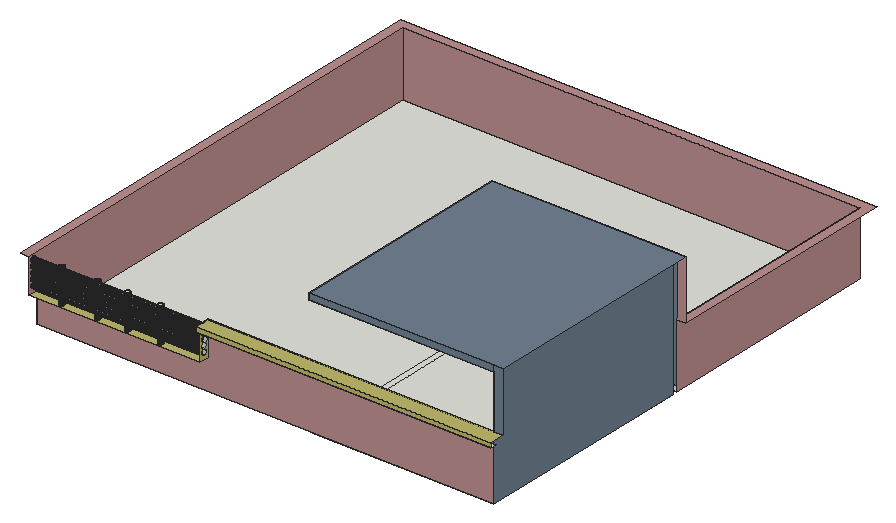
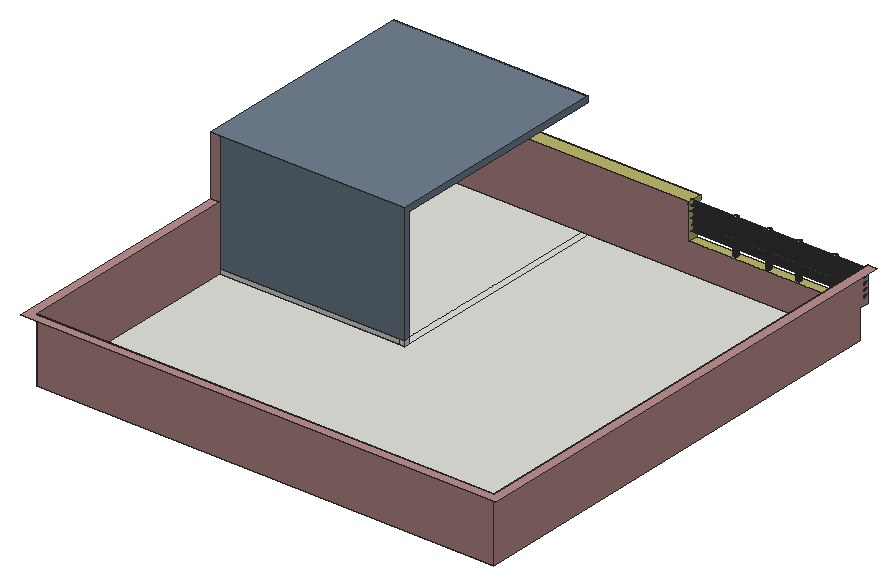
# SketchUp Ruby script. Lengths in inches.
U = 1.inch
M = Sketchup.active_model
def pt(a) = Geom::Point3d.new(a.map { |v| v * U })
def face(e, loops, mat)
  f = e.add_face(loops[0].map { |a| pt(a) })
  loops[1..].each { |l| e.add_face(l.map { |a| pt(a) }).erase! }
  f.material = f.back_material = mat if mat
  f
end
# faces: each face lists its corners as indices into pts; further lists are holes
def faces(e, pts, list, mat = nil) = list.each { |f| face(e, (f[0].is_a?(Array) ? f : [f]).map { |l| l.map { |i| pts[i] } }, mat) }
# xy, xz, yz: faces in a plane at the given z, y or x. An outline is a flat list of corners, or four numbers for a rectangle; further outlines are holes
def ring(l) = l.size == 4 ? [[l[0], l[1]], [l[2], l[1]], [l[2], l[3]], [l[0], l[3]]] : l.each_slice(2).to_a
def flat(e, list, mat, &to3) = list.each { |f| face(e, (f[0].is_a?(Array) ? f : [f]).map { |l| ring(l).map { |u, v| to3.(u, v) } }, mat) }
def xy(e, z, list, mat = nil) = flat(e, list, mat) { |x, y| [x, y, z] }
def xz(e, y, list, mat = nil) = flat(e, list, mat) { |x, z| [x, y, z] }
def yz(e, x, list, mat = nil) = flat(e, list, mat) { |y, z| [x, y, z] }
def lines(e, pts, list) = list.each { |a, b| e.add_line(pt(pts[a]), pt(pts[b])) }
# prism: a flat outline (further loops are holes) pulled along v
def prism(e, loops, v, mat = nil)
  f = face(e, loops, mat); d = Geom::Vector3d.new(v.map { |x| x * U })
  f.pushpull(f.normal.samedirection?(d) ? d.length : -d.length)
end
def box(e, o, s, mat = nil) = prism(e, [[o, [o[0] + s[0], o[1], o[2]], [o[0] + s[0], o[1] + s[1], o[2]], [o[0], o[1] + s[1], o[2]]]], [0, 0, s[2]], mat)
def at(x, y, z, deg = 0) = Geom::Transformation.translation(pt([x, y, z])) * Geom::Transformation.rotation(ORIGIN, Z_AXIS, deg.degrees)
def axes(o, x, y, z) = Geom::Transformation.new([*x, 0, *y, 0, *z, 0, *pt(o).to_a, 1])
def part(name) = M.definitions.add(name)
# library, detail: a bought-in or finely detailed component or shape, given as its bounding box
def library(name, o, s) = part(name).tap { |d| box(d.entities, o, s) }
def detail(e, o, s) = box(e.add_group.entities, o, s)
def put(e, d, t, mat = nil) = e.add_instance(d, t).tap { |i| i.material = mat if mat }
def group(e, t, mat = nil) = e.add_group.tap { |g| g.transformation = t; g.material = mat if mat }.entities
root = M.entities
M.materials.add("[0057_DarkKhaki]").color = [189, 183, 107]
M.materials.add("[0111_SlateGray]").color = [112, 128, 144]
M.materials.add("[0119_RosyBrown]").color = [188, 143, 143]
xy(root,486.9375,[[9,21,284.375,21,284.375,251.9375,471,251.9375,471,483,9,483],[284.375,21,290.375,245.9375],[290.375,21,471,245.9375]])
xy(root,517.1875,[[[9,12,181.625,21],[138.23,13.86,137.65,13.9375,137.11,14.16,136.64,14.52,136.28,14.99,136.06,15.53,135.98,16.11,136.06,16.69,136.28,17.24,136.64,17.7,137.11,18.06,137.65,18.28,138.23,18.36,138.81,18.28,139.36,18.06,139.82,17.7,140.18,17.24,140.41,16.69,140.48,16.11,140.41,15.53,140.18,14.99,139.82,14.52,139.36,14.16,138.81,13.9375],[38.67,13.86,38.09,13.9375,37.54,14.16,37.08,14.52,36.72,14.99,36.5,15.53,36.42,16.11,36.5,16.69,36.72,17.24,37.08,17.7,37.54,18.06,38.09,18.28,38.67,18.36,39.25,18.28,39.79,18.06,40.26,17.7,40.62,17.24,40.84,16.69,40.92,16.11,40.84,15.53,40.62,14.99,40.26,14.52,39.79,14.16,39.25,13.9375],[74.67,13.86,74.09,13.9375,73.54,14.16,73.08,14.52,72.72,14.99,72.5,15.53,72.42,16.11,72.5,16.69,72.72,17.24,73.08,17.7,73.54,18.06,74.09,18.28,74.67,18.36,75.25,18.28,75.79,18.06,76.26,17.7,76.62,17.24,76.84,16.69,76.92,16.11,76.84,15.53,76.62,14.99,76.26,14.52,75.79,14.16,75.25,13.9375],[104.92,13.86,104.34,13.9375,103.79,14.16,103.33,14.52,102.97,14.99,102.75,15.53,102.67,16.11,102.75,16.69,102.97,17.24,103.33,17.7,103.79,18.06,104.34,18.28,104.92,18.36,105.5,18.28,106.04,18.06,106.51,17.7,106.87,17.24,107.09,16.69,107.17,16.11,107.09,15.53,106.87,14.99,106.51,14.52,106.04,14.16,105.5,13.9375]]],"[0057_DarkKhaki]")
xy(root,547.59,[[181.625,5.9375,480,12]])
xy(root,552,[[181.625,5.9375,480,21]],"[0057_DarkKhaki]")
xy(root,552,[[0,12,9,12,9,483,471,483,471,251.9375,480,251.9375,480,492,0,492]],"[0119_RosyBrown]")
xy(root,552.3125,[[38.67,13.86,39.25,13.9375,39.79,14.16,40.26,14.52,40.62,14.99,40.84,15.53,40.92,16.11,40.84,16.69,40.62,17.24,40.26,17.7,39.79,18.06,39.25,18.28,38.67,18.36,38.09,18.28,37.54,18.06,37.08,17.7,36.72,17.24,36.5,16.69,36.42,16.11,36.5,15.53,36.72,14.99,37.08,14.52,37.54,14.16,38.09,13.9375],[74.67,13.86,75.25,13.9375,75.79,14.16,76.26,14.52,76.62,14.99,76.84,15.53,76.92,16.11,76.84,16.69,76.62,17.24,76.26,17.7,75.79,18.06,75.25,18.28,74.67,18.36,74.09,18.28,73.54,18.06,73.08,17.7,72.72,17.24,72.5,16.69,72.42,16.11,72.5,15.53,72.72,14.99,73.08,14.52,73.54,14.16,74.09,13.9375],[104.92,13.86,105.5,13.9375,106.04,14.16,106.51,14.52,106.87,14.99,107.09,15.53,107.17,16.11,107.09,16.69,106.87,17.24,106.51,17.7,106.04,18.06,105.5,18.28,104.92,18.36,104.34,18.28,103.79,18.06,103.33,17.7,102.97,17.24,102.75,16.69,102.67,16.11,102.75,15.53,102.97,14.99,103.33,14.52,103.79,14.16,104.34,13.9375],[138.23,13.86,138.81,13.9375,139.36,14.16,139.82,14.52,140.18,14.99,140.41,15.53,140.48,16.11,140.41,16.69,140.18,17.24,139.82,17.7,139.36,18.06,138.81,18.28,138.23,18.36,137.65,18.28,137.11,18.06,136.64,17.7,136.28,17.24,136.06,16.69,135.98,16.11,136.06,15.53,136.28,14.99,136.64,14.52,137.11,14.16,137.65,13.9375]])
xy(root,606,[[284.375,21,471,245.9375]],"[0111_SlateGray]")
xy(root,612,[[284.375,21,480,251.9375]],"[0111_SlateGray]")
xz(root,5.9375,[[181.625,547.59,480,552]],"[0057_DarkKhaki]")
xz(root,21,[[471,552,480,612],[284.375,606,471,612]],"[0111_SlateGray]")
xz(root,21,[[9,486.9375,9,517.1875,181.625,517.1875,181.625,552,471,552,471,486.9375]],"[0119_RosyBrown]")
xz(root,245.9375,[[284.375,486.9375,471,606]],"[0111_SlateGray]")
xz(root,251.9375,[[284.375,486.9375,290.375,492],[290.375,486.9375,471,492]])
xz(root,251.9375,[[284.375,492,471,612]],"[0111_SlateGray]")
xz(root,251.9375,[[471,552,480,612]],"[0119_RosyBrown]")
xz(root,483,[[9,486.9375,471,552]],"[0119_RosyBrown]")
yz(root,9,[[[21,486.9375,483,486.9375,483,552,12,552,12,517.1875,21,517.1875],[15.23,546.42,14.65,546.5,14.1,546.72,13.64,547.08,13.28,547.55,13.05,548.09,12.98,548.67,13.05,549.25,13.28,549.8,13.64,550.26,14.1,550.62,14.65,550.84,15.23,550.92,15.81,550.84,16.35,550.62,16.82,550.26,17.18,549.8,17.4,549.25,17.48,548.67,17.4,548.09,17.18,547.55,16.82,547.08,16.35,546.72,15.81,546.5],[15.23,540.55,14.65,540.62,14.1,540.85,13.64,541.2,13.28,541.67,13.05,542.21,12.98,542.8,13.05,543.38,13.28,543.92,13.64,544.39,14.1,544.74,14.65,544.97,15.23,545.05,15.81,544.97,16.35,544.74,16.82,544.39,17.18,543.92,17.4,543.38,17.48,542.8,17.4,542.21,17.18,541.67,16.82,541.2,16.35,540.85,15.81,540.62],[15.23,534.67,14.65,534.75,14.1,534.97,13.64,535.33,13.28,535.8,13.05,536.34,12.98,536.92,13.05,537.5,13.28,538.05,13.64,538.51,14.1,538.87,14.65,539.09,15.23,539.17,15.81,539.09,16.35,538.87,16.82,538.51,17.18,538.05,17.4,537.5,17.48,536.92,17.4,536.34,17.18,535.8,16.82,535.33,16.35,534.97,15.81,534.75],[15.23,528.8,14.65,528.87,14.1,529.1,13.64,529.45,13.28,529.92,13.05,530.46,12.98,531.05,13.05,531.63,13.28,532.17,13.64,532.64,14.1,532.99,14.65,533.22,15.23,533.3,15.81,533.22,16.35,532.99,16.82,532.64,17.18,532.17,17.4,531.63,17.48,531.05,17.4,530.46,17.18,529.92,16.82,529.45,16.35,529.1,15.81,528.87],[15.23,522.92,14.65,523,14.1,523.22,13.64,523.58,13.28,524.05,13.05,524.59,12.98,525.17,13.05,525.75,13.28,526.3,13.64,526.76,14.1,527.12,14.65,527.34,15.23,527.42,15.81,527.34,16.35,527.12,16.82,526.76,17.18,526.3,17.4,525.75,17.48,525.17,17.4,524.59,17.18,524.05,16.82,523.58,16.35,523.22,15.81,523]]],"[0119_RosyBrown]")
yz(root,181.625,[[12,517.1875,12,547.59,5.9375,547.59,5.9375,552,21,552,21,517.1875]],"[0057_DarkKhaki]")
yz(root,182.75,[[15.23,528.8,15.81,528.87,16.35,529.1,16.82,529.45,17.18,529.92,17.4,530.46,17.48,531.05,17.4,531.63,17.18,532.17,16.82,532.64,16.35,532.99,15.81,533.22,15.23,533.3,14.65,533.22,14.1,532.99,13.64,532.64,13.28,532.17,13.05,531.63,12.98,531.05,13.05,530.46,13.28,529.92,13.64,529.45,14.1,529.1,14.65,528.87]])
yz(root,183.0625,[[15.23,522.92,15.81,523,16.35,523.22,16.82,523.58,17.18,524.05,17.4,524.59,17.48,525.17,17.4,525.75,17.18,526.3,16.82,526.76,16.35,527.12,15.81,527.34,15.23,527.42,14.65,527.34,14.1,527.12,13.64,526.76,13.28,526.3,13.05,525.75,12.98,525.17,13.05,524.59,13.28,524.05,13.64,523.58,14.1,523.22,14.65,523]])
yz(root,183.875,[[15.23,534.67,15.81,534.75,16.35,534.97,16.82,535.33,17.18,535.8,17.4,536.34,17.48,536.92,17.4,537.5,17.18,538.05,16.82,538.51,16.35,538.87,15.81,539.09,15.23,539.17,14.65,539.09,14.1,538.87,13.64,538.51,13.28,538.05,13.05,537.5,12.98,536.92,13.05,536.34,13.28,535.8,13.64,535.33,14.1,534.97,14.65,534.75]])
yz(root,184.8125,[[15.23,540.55,15.81,540.62,16.35,540.85,16.82,541.2,17.18,541.67,17.4,542.21,17.48,542.8,17.4,543.38,17.18,543.92,16.82,544.39,16.35,544.74,15.81,544.97,15.23,545.05,14.65,544.97,14.1,544.74,13.64,544.39,13.28,543.92,13.05,543.38,12.98,542.8,13.05,542.21,13.28,541.67,13.64,541.2,14.1,540.85,14.65,540.62]])
yz(root,186.125,[[15.23,546.42,15.81,546.5,16.35,546.72,16.82,547.08,17.18,547.55,17.4,548.09,17.48,548.67,17.4,549.25,17.18,549.8,16.82,550.26,16.35,550.62,15.81,550.84,15.23,550.92,14.65,550.84,14.1,550.62,13.64,550.26,13.28,549.8,13.05,549.25,12.98,548.67,13.05,548.09,13.28,547.55,13.64,547.08,14.1,546.72,14.65,546.5]])
yz(root,284.375,[[245.9375,486.9375,251.9375,492]])
yz(root,284.375,[[245.9375,492,245.9375,606,21,606,21,612,251.9375,612,251.9375,492]],"[0111_SlateGray]")
yz(root,471,[[21,486.9375,245.9375,606]],"[0111_SlateGray]")
yz(root,471,[[251.9375,486.9375,483,552]],"[0119_RosyBrown]")
p = [[37.54,14.16,517.1875],[38.09,13.9375,517.1875],[38.09,13.9375,552.3125],[37.54,14.16,552.3125],[38.67,13.86,517.1875],[38.67,13.86,552.3125],
  [39.25,13.9375,517.1875],[39.25,13.9375,552.3125],[39.79,14.16,517.1875],[39.79,14.16,552.3125],[73.54,14.16,517.1875],[74.09,13.9375,517.1875],
  [74.09,13.9375,552.3125],[73.54,14.16,552.3125],[74.67,13.86,517.1875],[74.67,13.86,552.3125],[75.25,13.9375,517.1875],[75.25,13.9375,552.3125],
  [75.79,14.16,517.1875],[75.79,14.16,552.3125],[103.79,14.16,517.1875],[104.34,13.9375,517.1875],[104.34,13.9375,552.3125],[103.79,14.16,552.3125],
  [104.92,13.86,517.1875],[104.92,13.86,552.3125],[105.5,13.9375,517.1875],[105.5,13.9375,552.3125],[106.04,14.16,517.1875],[106.04,14.16,552.3125],
  [137.11,14.16,517.1875],[137.65,13.9375,517.1875],[137.65,13.9375,552.3125],[137.11,14.16,552.3125],[138.23,13.86,517.1875],[138.23,13.86,552.3125],
  [138.81,13.9375,517.1875],[138.81,13.9375,552.3125],[139.36,14.16,517.1875],[139.36,14.16,552.3125],[37.08,14.52,517.1875],[37.08,14.52,552.3125],
  [40.26,14.52,517.1875],[40.26,14.52,552.3125],[73.08,14.52,517.1875],[73.08,14.52,552.3125],[76.26,14.52,517.1875],[76.26,14.52,552.3125],
  [103.33,14.52,517.1875],[103.33,14.52,552.3125],[106.51,14.52,517.1875],[106.51,14.52,552.3125],[136.64,14.52,517.1875],[136.64,14.52,552.3125],
  [139.82,14.52,517.1875],[139.82,14.52,552.3125],[36.72,14.99,517.1875],[36.72,14.99,552.3125],[40.62,14.99,517.1875],[40.62,14.99,552.3125],
  [72.72,14.99,517.1875],[72.72,14.99,552.3125],[76.62,14.99,517.1875],[76.62,14.99,552.3125],[102.97,14.99,517.1875],[102.97,14.99,552.3125],
  [106.87,14.99,517.1875],[106.87,14.99,552.3125],[136.28,14.99,517.1875],[136.28,14.99,552.3125],[140.18,14.99,517.1875],[140.18,14.99,552.3125],
  [36.5,15.53,517.1875],[36.5,15.53,552.3125],[40.84,15.53,517.1875],[40.84,15.53,552.3125],[72.5,15.53,517.1875],[72.5,15.53,552.3125],
  [76.84,15.53,517.1875],[76.84,15.53,552.3125],[102.75,15.53,517.1875],[102.75,15.53,552.3125],[107.09,15.53,517.1875],[107.09,15.53,552.3125],
  [136.06,15.53,517.1875],[136.06,15.53,552.3125],[140.41,15.53,517.1875],[140.41,15.53,552.3125],[36.42,16.11,517.1875],[36.42,16.11,552.3125],
  [40.92,16.11,517.1875],[40.92,16.11,552.3125],[72.42,16.11,517.1875],[72.42,16.11,552.3125],[76.92,16.11,517.1875],[76.92,16.11,552.3125],
  [102.67,16.11,517.1875],[102.67,16.11,552.3125],[107.17,16.11,517.1875],[107.17,16.11,552.3125],[135.98,16.11,517.1875],[135.98,16.11,552.3125],
  [140.48,16.11,517.1875],[140.48,16.11,552.3125],[36.5,16.69,517.1875],[36.5,16.69,552.3125],[40.84,16.69,517.1875],[40.84,16.69,552.3125],
  [72.5,16.69,517.1875],[72.5,16.69,552.3125],[76.84,16.69,517.1875],[76.84,16.69,552.3125],[102.75,16.69,517.1875],[102.75,16.69,552.3125],
  [107.09,16.69,517.1875],[107.09,16.69,552.3125],[136.06,16.69,517.1875],[136.06,16.69,552.3125],[140.41,16.69,517.1875],[140.41,16.69,552.3125],
  [36.72,17.24,517.1875],[36.72,17.24,552.3125],[40.62,17.24,517.1875],[40.62,17.24,552.3125],[72.72,17.24,517.1875],[72.72,17.24,552.3125],
  [76.62,17.24,517.1875],[76.62,17.24,552.3125],[102.97,17.24,517.1875],[102.97,17.24,552.3125],[106.87,17.24,517.1875],[106.87,17.24,552.3125],
  [136.28,17.24,517.1875],[136.28,17.24,552.3125],[140.18,17.24,517.1875],[140.18,17.24,552.3125],[37.08,17.7,517.1875],[37.08,17.7,552.3125],
  [40.26,17.7,517.1875],[40.26,17.7,552.3125],[73.08,17.7,517.1875],[73.08,17.7,552.3125],[76.26,17.7,517.1875],[76.26,17.7,552.3125],
  [103.33,17.7,517.1875],[103.33,17.7,552.3125],[106.51,17.7,517.1875],[106.51,17.7,552.3125],[136.64,17.7,517.1875],[136.64,17.7,552.3125],
  [139.82,17.7,517.1875],[139.82,17.7,552.3125],[37.54,18.06,517.1875],[37.54,18.06,552.3125],[39.79,18.06,517.1875],[39.79,18.06,552.3125],
  [73.54,18.06,517.1875],[73.54,18.06,552.3125],[75.79,18.06,517.1875],[75.79,18.06,552.3125],[103.79,18.06,517.1875],[103.79,18.06,552.3125],
  [106.04,18.06,517.1875],[106.04,18.06,552.3125],[137.11,18.06,517.1875],[137.11,18.06,552.3125],[139.36,18.06,517.1875],[139.36,18.06,552.3125],
  [38.09,18.28,517.1875],[38.09,18.28,552.3125],[39.25,18.28,517.1875],[39.25,18.28,552.3125],[74.09,18.28,517.1875],[74.09,18.28,552.3125],
  [75.25,18.28,517.1875],[75.25,18.28,552.3125],[104.34,18.28,517.1875],[104.34,18.28,552.3125],[105.5,18.28,517.1875],[105.5,18.28,552.3125],
  [137.65,18.28,517.1875],[137.65,18.28,552.3125],[138.81,18.28,517.1875],[138.81,18.28,552.3125],[38.67,18.36,517.1875],[38.67,18.36,552.3125],
  [74.67,18.36,517.1875],[74.67,18.36,552.3125],[104.92,18.36,517.1875],[104.92,18.36,552.3125],[138.23,18.36,517.1875],[138.23,18.36,552.3125],
  [9,14.65,523],[9,15.23,522.92],[183.0625,15.23,522.92],[183.0625,14.65,523],[9,15.81,523],[183.0625,15.81,523],
  [9,14.1,523.22],[183.0625,14.1,523.22],[9,16.35,523.22],[183.0625,16.35,523.22],[9,13.64,523.58],[183.0625,13.64,523.58],
  [9,16.82,523.58],[183.0625,16.82,523.58],[9,13.28,524.05],[183.0625,13.28,524.05],[9,17.18,524.05],[183.0625,17.18,524.05],
  [9,13.05,524.59],[183.0625,13.05,524.59],[9,17.4,524.59],[183.0625,17.4,524.59],[9,12.98,525.17],[183.0625,12.98,525.17],
  [9,17.48,525.17],[183.0625,17.48,525.17],[9,13.05,525.75],[183.0625,13.05,525.75],[9,17.4,525.75],[183.0625,17.4,525.75],
  [9,13.28,526.3],[183.0625,13.28,526.3],[9,17.18,526.3],[183.0625,17.18,526.3],[9,13.64,526.76],[183.0625,13.64,526.76],
  [9,16.82,526.76],[183.0625,16.82,526.76],[9,14.1,527.12],[183.0625,14.1,527.12],[9,16.35,527.12],[183.0625,16.35,527.12],
  [9,14.65,527.34],[183.0625,14.65,527.34],[9,15.81,527.34],[183.0625,15.81,527.34],[9,15.23,527.42],[183.0625,15.23,527.42],
  [9,14.65,528.87],[9,15.23,528.8],[182.75,15.23,528.8],[182.75,14.65,528.87],[9,15.81,528.87],[182.75,15.81,528.87],
  [9,14.1,529.1],[182.75,14.1,529.1],[9,16.35,529.1],[182.75,16.35,529.1],[9,13.64,529.45],[182.75,13.64,529.45],
  [9,16.82,529.45],[182.75,16.82,529.45],[9,13.28,529.92],[182.75,13.28,529.92],[9,17.18,529.92],[182.75,17.18,529.92],
  [9,13.05,530.46],[182.75,13.05,530.46],[9,17.4,530.46],[182.75,17.4,530.46],[9,12.98,531.05],[182.75,12.98,531.05],
  [9,17.48,531.05],[182.75,17.48,531.05],[9,13.05,531.63],[182.75,13.05,531.63],[9,17.4,531.63],[182.75,17.4,531.63],
  [9,13.28,532.17],[182.75,13.28,532.17],[9,17.18,532.17],[182.75,17.18,532.17],[9,13.64,532.64],[182.75,13.64,532.64],
  [9,16.82,532.64],[182.75,16.82,532.64],[9,14.1,532.99],[182.75,14.1,532.99],[9,16.35,532.99],[182.75,16.35,532.99],
  [9,14.65,533.22],[182.75,14.65,533.22],[9,15.81,533.22],[182.75,15.81,533.22],[9,15.23,533.3],[182.75,15.23,533.3],
  [9,14.1,534.97],[9,14.65,534.75],[183.875,14.65,534.75],[183.875,14.1,534.97],[9,15.23,534.67],[183.875,15.23,534.67],
  [9,15.81,534.75],[183.875,15.81,534.75],[9,16.35,534.97],[183.875,16.35,534.97],[9,13.64,535.33],[183.875,13.64,535.33],
  [9,16.82,535.33],[183.875,16.82,535.33],[9,13.28,535.8],[183.875,13.28,535.8],[9,17.18,535.8],[183.875,17.18,535.8],
  [9,13.05,536.34],[183.875,13.05,536.34],[9,17.4,536.34],[183.875,17.4,536.34],[9,12.98,536.92],[183.875,12.98,536.92],
  [9,17.48,536.92],[183.875,17.48,536.92],[9,13.05,537.5],[183.875,13.05,537.5],[9,17.4,537.5],[183.875,17.4,537.5],
  [9,13.28,538.05],[183.875,13.28,538.05],[9,17.18,538.05],[183.875,17.18,538.05],[9,13.64,538.51],[183.875,13.64,538.51],
  [9,16.82,538.51],[183.875,16.82,538.51],[9,14.1,538.87],[183.875,14.1,538.87],[9,16.35,538.87],[183.875,16.35,538.87],
  [9,14.65,539.09],[183.875,14.65,539.09],[9,15.81,539.09],[183.875,15.81,539.09],[9,15.23,539.17],[183.875,15.23,539.17],
  [9,14.65,540.62],[9,15.23,540.55],[184.8125,15.23,540.55],[184.8125,14.65,540.62],[9,15.81,540.62],[184.8125,15.81,540.62],
  [9,14.1,540.85],[184.8125,14.1,540.85],[9,16.35,540.85],[184.8125,16.35,540.85],[9,13.64,541.2],[184.8125,13.64,541.2],
  [9,16.82,541.2],[184.8125,16.82,541.2],[9,13.28,541.67],[184.8125,13.28,541.67],[9,17.18,541.67],[184.8125,17.18,541.67],
  [9,13.05,542.21],[184.8125,13.05,542.21],[9,17.4,542.21],[184.8125,17.4,542.21],[9,12.98,542.8],[184.8125,12.98,542.8],
  [9,17.48,542.8],[184.8125,17.48,542.8],[9,13.05,543.38],[184.8125,13.05,543.38],[9,17.4,543.38],[184.8125,17.4,543.38],
  [9,13.28,543.92],[184.8125,13.28,543.92],[9,17.18,543.92],[184.8125,17.18,543.92],[9,13.64,544.39],[184.8125,13.64,544.39],
  [9,16.82,544.39],[184.8125,16.82,544.39],[9,14.1,544.74],[184.8125,14.1,544.74],[9,16.35,544.74],[184.8125,16.35,544.74],
  [9,14.65,544.97],[184.8125,14.65,544.97],[9,15.81,544.97],[184.8125,15.81,544.97],[9,15.23,545.05],[184.8125,15.23,545.05],
  [9,14.65,546.5],[9,15.23,546.42],[186.125,15.23,546.42],[186.125,14.65,546.5],[9,15.81,546.5],[186.125,15.81,546.5],
  [9,14.1,546.72],[186.125,14.1,546.72],[9,16.35,546.72],[186.125,16.35,546.72],[9,13.64,547.08],[186.125,13.64,547.08],
  [9,16.82,547.08],[186.125,16.82,547.08],[9,13.28,547.55],[186.125,13.28,547.55],[9,17.18,547.55],[186.125,17.18,547.55],
  [9,13.05,548.09],[186.125,13.05,548.09],[9,17.4,548.09],[186.125,17.4,548.09],[9,12.98,548.67],[186.125,12.98,548.67],
  [9,17.48,548.67],[186.125,17.48,548.67],[9,13.05,549.25],[186.125,13.05,549.25],[9,17.4,549.25],[186.125,17.4,549.25],
  [9,13.28,549.8],[186.125,13.28,549.8],[9,17.18,549.8],[186.125,17.18,549.8],[9,13.64,550.26],[186.125,13.64,550.26],
  [9,16.82,550.26],[186.125,16.82,550.26],[9,14.1,550.62],[186.125,14.1,550.62],[9,16.35,550.62],[186.125,16.35,550.62],
  [9,14.65,550.84],[186.125,14.65,550.84],[9,15.81,550.84],[186.125,15.81,550.84],[9,15.23,550.92],[186.125,15.23,550.92],
  [471,245.9375,492],[471,251.9375,492],[471,245.9375,606],[471,245.9375,612]]
faces(root,p,[[0,1,2,3],[1,4,5,2],[4,6,7,5],[6,8,9,7],[10,11,12,13],[11,14,15,12],[14,16,17,15],[16,18,19,17],
  [20,21,22,23],[21,24,25,22],[24,26,27,25],[26,28,29,27],[30,31,32,33],[31,34,35,32],[34,36,37,35],[36,38,39,37],
  [40,0,3,41],[8,42,43,9],[44,10,13,45],[18,46,47,19],[48,20,23,49],[28,50,51,29],[52,30,33,53],[38,54,55,39],
  [56,40,41,57],[42,58,59,43],[60,44,45,61],[46,62,63,47],[64,48,49,65],[50,66,67,51],[68,52,53,69],[54,70,71,55],
  [72,56,57,73],[58,74,75,59],[76,60,61,77],[62,78,79,63],[80,64,65,81],[66,82,83,67],[84,68,69,85],[70,86,87,71],
  [88,72,73,89],[74,90,91,75],[92,76,77,93],[78,94,95,79],[96,80,81,97],[82,98,99,83],[100,84,85,101],[86,102,103,87],
  [104,88,89,105],[90,106,107,91],[108,92,93,109],[94,110,111,95],[112,96,97,113],[98,114,115,99],[116,100,101,117],[102,118,119,103],
  [120,104,105,121],[106,122,123,107],[124,108,109,125],[110,126,127,111],[128,112,113,129],[114,130,131,115],[132,116,117,133],[118,134,135,119],
  [136,120,121,137],[122,138,139,123],[140,124,125,141],[126,142,143,127],[144,128,129,145],[130,146,147,131],[148,132,133,149],[134,150,151,135],
  [152,136,137,153],[138,154,155,139],[156,140,141,157],[142,158,159,143],[160,144,145,161],[146,162,163,147],[164,148,149,165],[150,166,167,151],
  [168,152,153,169],[154,170,171,155],[172,156,157,173],[158,174,175,159],[176,160,161,177],[162,178,179,163],[180,164,165,181],[166,182,183,167],
  [184,168,169,185],[170,184,185,171],[186,172,173,187],[174,186,187,175],[188,176,177,189],[178,188,189,179],[190,180,181,191],[182,190,191,183],
  [192,193,194,195],[193,196,197,194],[198,192,195,199],[196,200,201,197],[202,198,199,203],[200,204,205,201],[206,202,203,207],[204,208,209,205],
  [210,206,207,211],[208,212,213,209],[214,210,211,215],[212,216,217,213],[218,214,215,219],[216,220,221,217],[222,218,219,223],[220,224,225,221],
  [226,222,223,227],[224,228,229,225],[230,226,227,231],[228,232,233,229],[234,230,231,235],[232,236,237,233],[238,234,235,239],[236,238,239,237],
  [240,241,242,243],[241,244,245,242],[246,240,243,247],[244,248,249,245],[250,246,247,251],[248,252,253,249],[254,250,251,255],[252,256,257,253],
  [258,254,255,259],[256,260,261,257],[262,258,259,263],[260,264,265,261],[266,262,263,267],[264,268,269,265],[270,266,267,271],[268,272,273,269],
  [274,270,271,275],[272,276,277,273],[278,274,275,279],[276,280,281,277],[282,278,279,283],[280,284,285,281],[286,282,283,287],[284,286,287,285],
  [288,289,290,291],[289,292,293,290],[292,294,295,293],[294,296,297,295],[298,288,291,299],[296,300,301,297],[302,298,299,303],[300,304,305,301],
  [306,302,303,307],[304,308,309,305],[310,306,307,311],[308,312,313,309],[314,310,311,315],[312,316,317,313],[318,314,315,319],[316,320,321,317],
  [322,318,319,323],[320,324,325,321],[326,322,323,327],[324,328,329,325],[330,326,327,331],[328,332,333,329],[334,330,331,335],[332,334,335,333],
  [336,337,338,339],[337,340,341,338],[342,336,339,343],[340,344,345,341],[346,342,343,347],[344,348,349,345],[350,346,347,351],[348,352,353,349],
  [354,350,351,355],[352,356,357,353],[358,354,355,359],[356,360,361,357],[362,358,359,363],[360,364,365,361],[366,362,363,367],[364,368,369,365],
  [370,366,367,371],[368,372,373,369],[374,370,371,375],[372,376,377,373],[378,374,375,379],[376,380,381,377],[382,378,379,383],[380,382,383,381],
  [384,385,386,387],[385,388,389,386],[390,384,387,391],[388,392,393,389],[394,390,391,395],[392,396,397,393],[398,394,395,399],[396,400,401,397],
  [402,398,399,403],[400,404,405,401],[406,402,403,407],[404,408,409,405],[410,406,407,411],[408,412,413,409],[414,410,411,415],[412,416,417,413],
  [418,414,415,419],[416,420,421,417],[422,418,419,423],[420,424,425,421],[426,422,423,427],[424,428,429,425],[430,426,427,431],[428,430,431,429]],"[0111_SlateGray]")
lines(root,p,[[432,433],[434,435]])
